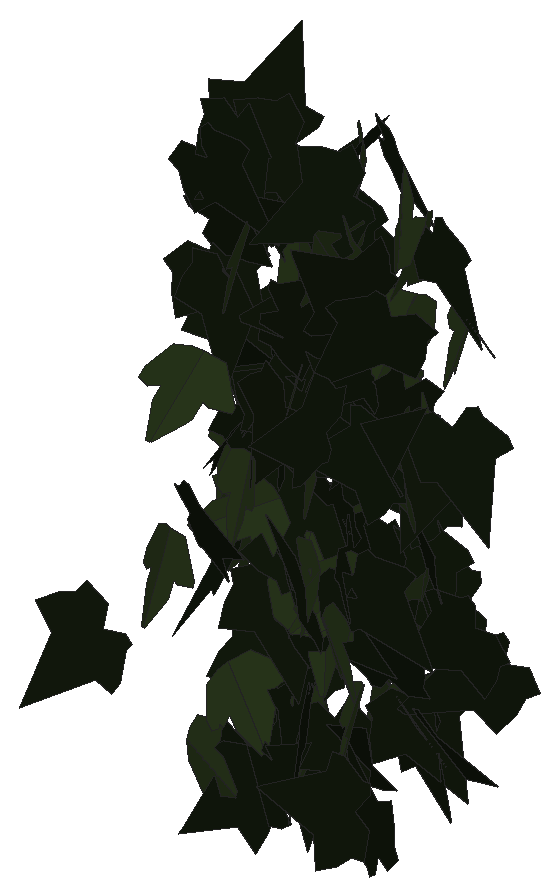
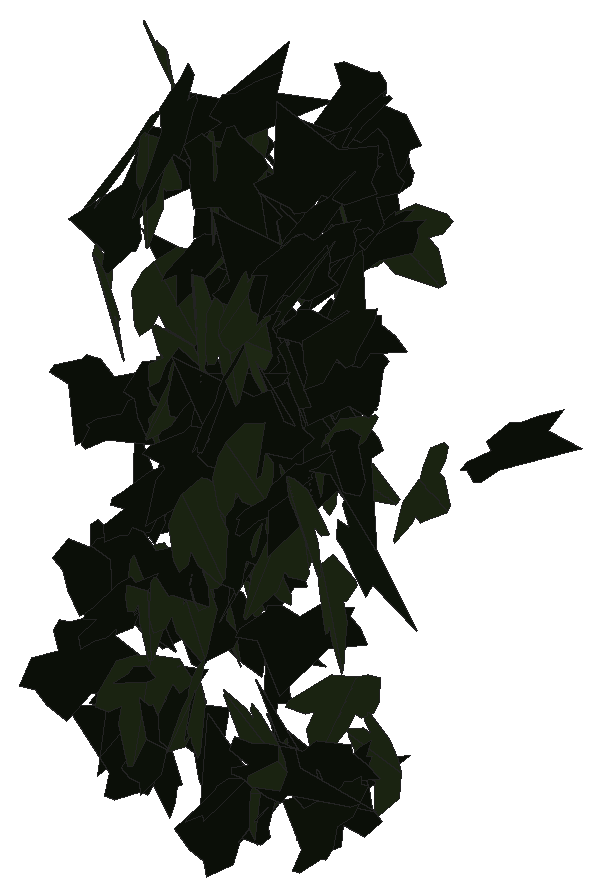
# SketchUp Ruby script. Lengths in inches.
U = 1.inch
M = Sketchup.active_model
def pt(a) = Geom::Point3d.new(a.map { |v| v * U })
def face(e, loops, mat)
  f = e.add_face(loops[0].map { |a| pt(a) })
  loops[1..].each { |l| e.add_face(l.map { |a| pt(a) }).erase! }
  f.material = f.back_material = mat if mat
  f
end
# faces: each face lists its corners as indices into pts; further lists are holes
def faces(e, pts, list, mat = nil) = list.each { |f| face(e, (f[0].is_a?(Array) ? f : [f]).map { |l| l.map { |i| pts[i] } }, mat) }
# xy, xz, yz: faces in a plane at the given z, y or x. An outline is a flat list of corners, or four numbers for a rectangle; further outlines are holes
def ring(l) = l.size == 4 ? [[l[0], l[1]], [l[2], l[1]], [l[2], l[3]], [l[0], l[3]]] : l.each_slice(2).to_a
def flat(e, list, mat, &to3) = list.each { |f| face(e, (f[0].is_a?(Array) ? f : [f]).map { |l| ring(l).map { |u, v| to3.(u, v) } }, mat) }
def xy(e, z, list, mat = nil) = flat(e, list, mat) { |x, y| [x, y, z] }
def xz(e, y, list, mat = nil) = flat(e, list, mat) { |x, z| [x, y, z] }
def yz(e, x, list, mat = nil) = flat(e, list, mat) { |y, z| [x, y, z] }
def lines(e, pts, list) = list.each { |a, b| e.add_line(pt(pts[a]), pt(pts[b])) }
# prism: a flat outline (further loops are holes) pulled along v
def prism(e, loops, v, mat = nil)
  f = face(e, loops, mat); d = Geom::Vector3d.new(v.map { |x| x * U })
  f.pushpull(f.normal.samedirection?(d) ? d.length : -d.length)
end
def box(e, o, s, mat = nil) = prism(e, [[o, [o[0] + s[0], o[1], o[2]], [o[0] + s[0], o[1] + s[1], o[2]], [o[0], o[1] + s[1], o[2]]]], [0, 0, s[2]], mat)
def at(x, y, z, deg = 0) = Geom::Transformation.translation(pt([x, y, z])) * Geom::Transformation.rotation(ORIGIN, Z_AXIS, deg.degrees)
def axes(o, x, y, z) = Geom::Transformation.new([*x, 0, *y, 0, *z, 0, *pt(o).to_a, 1])
def part(name) = M.definitions.add(name)
# library, detail: a bought-in or finely detailed component or shape, given as its bounding box
def library(name, o, s) = part(name).tap { |d| box(d.entities, o, s) }
def detail(e, o, s) = box(e.add_group.entities, o, s)
def put(e, d, t, mat = nil) = e.add_instance(d, t).tap { |i| i.material = mat if mat }
def group(e, t, mat = nil) = e.add_group.tap { |g| g.transformation = t; g.material = mat if mat }.entities
root = M.entities
M.materials.add("efeu1").color = [18, 25, 13]
M.materials.add("efeu2").color = [43, 57, 29]
c1 = part("ivyleaf_10")
p = [[0,0.5,-0.03],[-0.0625,2.02,-0.43],[-0.19,2.01,-0.46],[-0.54,1.05,-0.29],[-0.52,0.625,-0.18],[-0.83,0.76,-0.28],
  [-1.16,0.64,-0.33],[-1.15,0.33,-0.24],[-0.77,-0.39,0.02],[-0.3,-0.51,0.16],[0.04,-0.48,0.23],[-0.02,2.01,-0.4375],
  [-0.06,2.01,-0.43],[0.04,-0.49,0.23],[0.67,-0.49,0.14],[1.38,0.36,-0.2],[1.375,0.51,-0.24],[0.81,0.65,-0.19],
  [0.62,0.59,-0.15],[0.6,1.09,-0.28],[0.5,1.23,-0.31]]
faces(c1.entities,p,[[0,1,2,3,4,5,6,7,8,9,10],[11,12,0,13,14,15,16,17,18,19,20]],"efeu2")
c2 = part("ivyleaf_9")
p = [[1.54,2.16,1.25],[1.36,2.04,1.19],[-0.21,0.99,0.68],[-0.71,1.11,0.82],[-0.85,0.86,0.67],[-0.8,0.17,0.21],
  [-0.9,-0.01,0.1],[-0.67,-0.16,-0.02],[-0.08,-0.08,-0.05],[-0.03,-0.6,-0.4],[0.65,-0.88,-0.66],[0.83,-0.6,-0.49],
  [1.29,-0.42,-0.43],[1.8125,-0.07,-0.26],[1.21,0.44,0.15]]
faces(c2.entities,p,[[0,1,2,3,4,5,6,7,8,9,10,11,12,13,14]],"efeu1")
put(root,c1,axes([32.31,222.57,218.74],[0.42395,-0.25551,-0.07061],[-0.0561,0.04368,-0.49492],[0.25908,0.42756,0.00837]))
put(root,c2,axes([32.14,222.04,220.38],[0.40377,-0.26731,-0.12456],[0.10558,-0.06616,0.48423],[-0.27536,-0.41734,0.00302]))
put(root,c2,axes([32.25,222.2,222.53],[-0.31553,-0.10498,0.37339],[0.37174,0.05553,0.32974],[-0.1107,0.48569,0.043]))
put(root,c2,axes([31.98,222.29,214.44],[0.21673,-0.35207,0.2812],[0.19342,-0.20914,-0.41092],[0.40696,0.28689,0.04554]))
put(root,c2,axes([32.16,222.17,222.4375],[0.07076,-0.49493,-0.00612],[-0.00103,0.00604,-0.49996],[0.49497,0.07077,-0.00016]))
put(root,c1,axes([32.39,221.875,217.21],[0.17943,-0.46368,-0.05301],[-0.01066,0.05271,-0.4971],[0.46658,0.17952,0.00903]))
put(root,c2,axes([32.23,222.39,221.93],[0.08557,-0.40622,-0.27869],[-0.00917,0.2815,-0.41313],[0.49254,0.07582,0.04072]))
put(root,c2,axes([32.81,222.71,215.1],[-0.40746,0.01612,0.28934],[-0.28964,-0.00698,-0.4075],[-0.0091,-0.49969,0.01503]))
put(root,c2,axes([32.39,222.33,215.23],[-0.29931,-0.3482,-0.19791],[0.138,0.14228,-0.45903],[0.37599,-0.32941,0.01094]))
put(root,c2,axes([32.67,221.375,218.97],[-0.19348,0.45479,-0.07573],[0.03096,-0.06913,-0.49423],[-0.46001,-0.19593,-0.00141]))
put(root,c1,axes([32.5,220.06,217.7],[0.00601,0.3694,-0.3369],[-0.01379,-0.33668,-0.3694],[-0.49977,0.01374,0.00614]))
put(root,c1,axes([32.52,221.59,218.74],[0.02832,-0.40737,0.28853],[0.10403,-0.27783,-0.40248],[0.48824,0.08283,0.06902]))
put(root,c2,axes([32.3,222.3,221.5],[0.26872,-0.4191,0.04638],[0.02591,-0.03848,-0.49784],[0.42086,0.26996,0.00104]))
put(root,c2,axes([32.74,221.02,217.41],[-0.38451,0.23721,-0.21419],[0.1678,-0.13536,-0.45113],[-0.27202,-0.41882,0.02448]))
put(root,c2,axes([32.52,221.64,220.46],[-0.28739,-0.3412,-0.2258],[0.14796,0.17059,-0.4461],[0.38146,-0.32323,0.00292]))
put(root,c2,axes([32.41,221.55,222.97],[0.10522,-0.48799,-0.02811],[-0.00403,0.02789,-0.49921],[0.48879,0.10528,0.00194]))
put(root,c2,axes([32.42,221.02,221.34],[0.09643,-0.3928,-0.29395],[0.0414,0.30502,-0.39402],[0.48886,0.05164,0.09135]))
put(root,c2,axes([32.79,222.09,222.54],[-0.27331,-0.26526,0.32394],[-0.19453,-0.2621,-0.37876],[0.37075,-0.33307,0.04007]))
put(root,c2,axes([32.74,218.43,217.34],[-0.25405,-0.35079,0.24981],[-0.12884,-0.21485,-0.43272],[0.41092,-0.28423,0.01878]))
put(root,c2,axes([32.65,221.7,218.95],[0.32197,0.38223,-0.01537],[-0.01291,-0.00921,-0.49975],[-0.38232,0.3222,0.00394]))
put(root,c2,axes([32.62,222.67,218.64],[-0.11973,-0.44473,0.19464],[-0.04975,-0.18817,-0.46056],[0.4829,-0.12966,0.00081]))
put(root,c1,axes([32.36,220.875,214.47],[-0.0658,0.03506,-0.49441],[0.38456,-0.31105,-0.07324],[-0.31271,-0.3899,0.01397]))
put(root,c2,axes([32.63,221.2,219.87],[0.38078,0.30351,0.11352],[0.08986,0.06939,-0.48694],[-0.31134,0.39123,-0.00171]))
put(root,c1,axes([32.7,221.16,215.42],[0.16282,0.44771,0.15182],[0.05846,0.14027,-0.47635],[-0.46912,0.17287,-0.00667]))
put(root,c2,axes([32.68,222.38,221.16],[-0.25046,-0.03882,0.431],[0.42418,0.07655,0.25339],[-0.08566,0.49258,-0.00541]))
put(root,c2,axes([32.49,220.79,222.9],[-0.03863,-0.0412,-0.4968],[0.42177,0.26292,-0.0546],[0.26574,-0.42329,0.01444]))
put(root,c2,axes([32.68,220.99,221.08],[0.02357,-0.49467,0.0689],[0.00007,-0.06897,-0.49522],[0.49944,0.02335,-0.00318]))
put(root,c2,axes([32.46,221.01,221.875],[0.41676,0.08791,-0.26188],[0.21045,0.20601,0.40407],[0.17895,-0.44702,0.13471]))
put(root,c1,axes([32.52,222.78,215.36],[0.13292,-0.09911,-0.47171],[0.39947,-0.25118,0.16533],[-0.26974,-0.42082,0.01241]))
put(root,c1,axes([32.87,222.9375,219.17],[-0.05063,-0.40683,0.28623],[0.09792,-0.29023,-0.39519],[0.4877,0.01604,0.10906]))
put(root,c2,axes([32.87,221.27,214.07],[0.10576,-0.22487,-0.43388],[0.18999,-0.39008,0.24848],[-0.45024,-0.21742,0.00294]))
put(root,c2,axes([32.76,221.72,214.36],[-0.19706,0.29241,0.35449],[0.20982,-0.2859,0.35247],[0.40883,0.28768,-0.01003]))
put(root,c1,axes([32.9,222.95,220.95],[-0.11769,0.21611,0.43525],[0.15057,-0.40958,0.24407],[0.46204,0.18852,0.03133]))
put(root,c2,axes([33.17,221.32,219.67],[-0.31568,0.37174,-0.11028],[0.07145,-0.08401,-0.48769],[-0.38111,-0.32366,-0.00008]))
put(root,c2,axes([32.6875,221.3,213.82],[-0.10946,0.06519,0.4835],[0.39718,-0.27584,0.12711],[0.28331,0.4119,0.00861]))
put(root,c1,axes([32.95,220.97,221.85],[0.26181,-0.40818,0.12186],[0.06481,-0.1032,-0.48492],[0.42102,0.26971,-0.00113]))
put(root,c1,axes([33.28,220.89,218.21],[0.25599,0.03919,-0.42771],[-0.4265,-0.03557,-0.25853],[-0.05069,0.49719,0.01521]))
put(root,c2,axes([33.37,222.06,219.75],[-0.28091,0.07538,-0.40671],[-0.40972,0.01678,0.28609],[0.05678,0.494,0.05234]))
put(root,c2,axes([33.16,221.37,218.43],[0.07392,-0.04564,0.4924],[-0.07408,0.49123,0.05665],[-0.48893,-0.08133,0.06586]))
put(root,c2,axes([32.89,221.78,216.5625],[-0.17419,-0.38433,-0.26823],[0.11242,0.24355,-0.42196],[0.45499,-0.20731,0.00156]))
put(root,c1,axes([33.04,221.94,217.66],[-0.02961,-0.35779,-0.34801],[0.06373,0.34305,-0.35812],[0.49504,-0.06557,0.02528]))
put(root,c1,axes([33.17,219.71,220.58],[0.32097,0.28919,-0.25169],[-0.18565,-0.16996,-0.43203],[-0.33543,0.37079,-0.00173]))
put(root,c2,axes([32.82,222.56,219.15],[-0.10704,-0.01487,0.48818],[0.48028,-0.09402,0.10244],[0.08875,0.49086,0.03441]))
put(root,c1,axes([33.01,222.33,214.49],[-0.00134,-0.22121,0.4484],[0.26873,-0.37845,-0.1859],[0.42164,0.2405,0.11991]))
put(root,c1,axes([33.24,222.66,220.74],[0.02883,-0.49844,-0.02702],[0.00013,0.02708,-0.49927],[0.49917,0.02878,0.00169]))
put(root,c2,axes([32.96,221.12,219.38],[0.04144,0.01784,-0.49796],[0.19221,0.46043,0.03249],[0.45971,-0.19412,0.03131]))
put(root,c1,axes([33.06,222.41,220.36],[0.17276,-0.21031,0.41943],[0.27027,-0.32076,-0.27216],[0.38355,0.32075,0.00285]))
put(root,c2,axes([33.05,222.09,214.25],[0.07021,-0.47379,0.1435],[0.01954,-0.14217,-0.47896],[0.49466,0.07287,-0.00144]))
put(root,c2,axes([33.125,222.98,219.84],[0.14798,-0.14163,-0.45612],[0.34089,-0.30312,0.20472],[-0.3345,-0.37157,0.00685]))
put(root,c2,axes([33.56,222.35,222.61],[-0.21193,0.42636,-0.15265],[0.04814,-0.14637,-0.47567],[-0.4503,-0.21632,0.02099]))
put(root,c1,axes([33.15,221.76,221.23],[0.31977,-0.13647,0.35933],[0.33699,-0.12529,-0.34747],[0.18489,0.46441,0.01185]))
put(root,c2,axes([33.4375,221.26,219.4],[-0.3062,-0.19412,0.34433],[0.31058,0.15127,0.36147],[-0.24451,0.43524,0.02794]))
put(root,c2,axes([33.78,222.56,219.21],[0.04114,-0.00309,0.4983],[-0.47583,0.14823,0.0402],[-0.14797,-0.47751,0.00926]))
put(root,c2,axes([33.1875,222.39,217.54],[0.0497,-0.17552,0.46553],[0.18697,-0.42697,-0.18094],[0.46106,0.19207,0.0232]))
put(root,c2,axes([33.2,222.5,214],[0.48721,-0.04367,-0.10352],[0.10669,0.0354,0.4872],[-0.03522,-0.49683,0.04381]))
put(root,c2,axes([33.33,222.3,214.55],[0.07332,-0.47465,-0.13904],[-0.00083,0.14044,-0.47987],[0.49459,0.0706,0.01981]))
put(root,c1,axes([33.59,221.29,220.23],[0.28433,-0.40044,-0.09383],[-0.04158,0.0855,-0.49088],[0.40918,0.28695,0.01532]))
put(root,c2,axes([33.83,221.67,217.66],[0.06786,-0.08371,0.48825],[-0.29047,0.39247,0.10766],[-0.40127,-0.29826,0.00463]))
put(root,c1,axes([33.7,222.33,222.5],[0.17303,-0.29338,-0.36604],[-0.13695,0.34156,-0.3385],[0.44867,0.2174,0.03784]))
put(root,c2,axes([33.46,221.46,217.53],[0.28464,-0.29456,-0.28674],[-0.18888,0.21605,-0.40945],[0.36511,0.34141,0.01172]))
put(root,c2,axes([33.82,221.25,217.57],[-0.37351,-0.32309,0.07815],[0.0608,0.04916,0.49385],[-0.3268,0.37842,0.00256]))
put(root,c1,axes([33.69,222.71,218.0625],[-0.00727,-0.46456,0.18474],[0.02734,-0.18486,-0.46377],[0.4992,0.00336,0.02809]))
put(root,c2,axes([33.9,222.48,218.6875],[-0.08354,-0.059,0.48943],[-0.40051,-0.2813,-0.10227],[0.28742,-0.40913,-0.00027]))
put(root,c2,axes([33.57,222.54,218.91],[-0.02965,-0.31912,-0.38377],[0.10077,0.37271,-0.31771],[0.48884,-0.09619,0.04221]))
put(root,c1,axes([33.92,222.35,220.7],[0.16493,-0.37373,-0.28832],[-0.11145,0.26594,-0.40848],[0.45867,0.19901,0.00442]))
put(root,c2,axes([34.23,221.16,221.14],[-0.09751,-0.09507,-0.4811],[-0.3884,-0.2845,0.13494],[-0.2994,0.40003,-0.01837]))
put(root,c2,axes([33.6,222.01,221.98],[-0.16548,-0.17035,-0.44],[0.39379,0.20697,-0.22823],[0.25989,-0.42207,0.06566]))
put(root,c1,axes([33.8,221.05,216.83],[0.49694,0.05359,-0.01355],[0.0134,0.00209,0.49982],[0.05363,-0.49712,0.00064]))
put(root,c2,axes([33.74,220.77,219.76],[-0.02738,-0.3822,0.32121],[-0.02304,-0.32038,-0.38318],[0.49872,-0.03579,-0.00006]))
put(root,c1,axes([33.97,222.28,215.42],[0.03969,-0.09222,-0.48982],[-0.0581,0.48716,-0.09643],[0.49502,0.06457,0.02795]))
put(root,c2,axes([33.75,222.25,221.42],[0.10763,-0.45316,-0.18182],[-0.04151,0.17702,-0.46577],[0.48651,0.11535,0.00048]))
put(root,c2,axes([34.11,221.58,222.51],[-0.24259,-0.25155,0.3576],[-0.24036,-0.26488,-0.34938],[0.36521,-0.34142,0.00759]))
put(root,c2,axes([33.83,221.12,215.49],[-0.16354,0.09011,-0.46383],[0.42072,-0.19564,-0.18634],[-0.21507,-0.45123,-0.01183]))
put(root,c1,axes([34.26,221.44,221.93],[-0.35349,0.06178,0.34817],[-0.34555,0.04417,-0.35867],[-0.07507,-0.4942,0.01147]))
put(root,c1,axes([34.15,220.78,217.57],[0.24726,-0.29081,-0.32294],[-0.20999,0.24535,-0.38172],[0.38048,0.3244,-0.00081]))
put(root,c2,axes([34.09,220.91,217.01],[0.13871,-0.42886,0.21642],[-0.02741,0.21783,0.44922],[-0.47959,-0.13649,0.03693]))
put(root,c2,axes([33.59,220.9375,220.98],[0.19162,-0.01967,-0.46141],[0.39057,0.27347,0.15055],[0.24644,-0.41812,0.12017]))
put(root,c1,axes([33.94,219.72,219.41],[0.41322,-0.26508,0.09477],[0.08082,-0.04953,-0.49093],[0.26966,0.42104,0.00192]))
put(root,c1,axes([34.17,222.3,219.48],[0.03638,-0.14598,-0.47683],[-0.01439,0.47759,-0.14731],[0.49847,0.02444,0.03055]))
put(root,c1,axes([33.96,221.26,216.78],[0.46324,-0.09978,0.15954],[0.15524,-0.03694,-0.47385],[0.10634,0.48855,-0.00324]))
put(root,c1,axes([34.08,221.38,221.65],[-0.08067,-0.37345,-0.32253],[-0.0126,-0.32515,0.37963],[-0.49329,0.06938,0.04305]))
put(root,c1,axes([33.83,222.52,219.72],[0.28334,0.0399,0.41003],[0.39739,0.10472,-0.2848],[-0.10861,0.48728,0.02763]))
put(root,c2,axes([33.83,221.125,216.93],[0.0591,-0.02817,-0.4957],[0.40425,0.29255,0.03157],[0.28825,-0.4045,0.05735]))
put(root,c2,axes([34.26,221.41,217.72],[0.20083,-0.1407,-0.43574],[-0.34872,0.26137,-0.24512],[0.29676,0.40235,0.00685]))
put(root,c1,axes([34.3,222.18,216.76],[-0.11806,-0.47316,0.11038],[-0.0201,-0.10874,-0.48762],[0.48545,-0.11957,0.00666]))
put(root,c2,axes([34.39,222.99,218.02],[-0.01171,-0.37473,-0.33082],[-0.00935,-0.33069,0.37491],[-0.49978,0.01497,0.00074]))
put(root,c1,axes([34.42,221.37,217.33],[0.23199,0.1961,-0.39715],[-0.29803,-0.26254,-0.30372],[-0.32765,0.37765,-0.00493]))
put(root,c2,axes([34.1,221.71,220.25],[-0.04526,-0.30569,0.39307],[0.0491,-0.39551,-0.30193],[0.49552,0.01127,0.06582]))
put(root,c2,axes([34.2,222.23,222.97],[0.39088,-0.15568,-0.27014],[-0.24935,0.10397,-0.42073],[0.18717,0.46363,0.00364]))
put(root,c1,axes([34.1,222.06,216.86],[-0.05364,0.04323,0.49523],[0.30389,-0.39135,0.06708],[0.39341,0.30819,0.01571]))
put(root,c2,axes([34.41,222.25,219.57],[-0.04171,0.14428,-0.47691],[0.13304,-0.45798,-0.15019],[-0.48017,-0.13943,-0.00018]))
put(root,c1,axes([34.4,222.35,220.68],[-0.17357,-0.40716,0.23258],[0.01817,-0.25365,-0.4305],[0.46856,-0.14099,0.10285]))
put(root,c2,axes([34.35,222.32,217.07],[-0.14554,-0.20553,0.43194],[-0.04227,-0.4442,-0.2256],[0.47648,-0.10219,0.11192]))
put(root,c2,axes([34.5,221.85,215.84],[0.34238,-0.16847,0.32311],[-0.28135,0.15953,0.38131],[-0.23157,-0.44291,0.01445]))
put(root,c2,axes([34.12,222.67,214.9],[0.38713,-0.11578,-0.29449],[0.28137,-0.08694,0.40407],[-0.14477,-0.47858,-0.00216]))
put(root,c1,axes([34.34,220.8,219.59],[0.1682,-0.37429,0.28569],[0.17293,-0.23306,-0.40716],[0.43795,0.23578,0.05105]))
put(root,c1,axes([34.375,222.17,218.5625],[0.16129,-0.45177,-0.14102],[0.04778,-0.13268,0.4797],[-0.47085,-0.16821,0.00037]))
put(root,c1,axes([34.57,222.41,216.89],[0.02054,-0.48637,-0.11413],[-0.00976,0.11382,-0.48678],[0.49948,0.02222,-0.00482]))
put(root,c2,axes([34.34,222.58,217.26],[-0.19721,-0.246,-0.38806],[0.26026,0.28821,-0.31496],[0.37865,-0.32622,0.01437]))
put(root,c2,axes([34.27,222.625,214.86],[-0.08518,-0.04186,-0.49091],[0.48583,0.07574,-0.09076],[0.08196,-0.49246,0.02777]))
put(root,c1,axes([34.63,222.36,215.44],[-0.32174,-0.37256,-0.08767],[0.05604,0.06744,-0.49225],[0.37861,-0.32658,-0.00164]))
put(root,c2,axes([34.79,222.98,216.46],[0.01335,-0.4207,-0.26987],[0.00931,-0.26971,0.42091],[-0.49973,-0.01627,0.00063]))
put(root,c2,axes([34.79,220.87,221.57],[0.11067,0.10687,0.47574],[-0.37505,-0.29309,0.15309],[0.31159,-0.39074,0.01529]))
put(root,c2,axes([34.92,221.11,213.86],[0.10325,-0.08462,0.48185],[-0.2244,0.42941,0.12349],[-0.43473,-0.24175,0.05069]))
put(root,c1,axes([34.66,221,215.86],[0.30377,-0.36777,0.14991],[0.09643,-0.11478,-0.477],[0.38526,0.3187,0.00119]))
put(root,c2,axes([34.62,222.24,215.33],[-0.01406,-0.34104,-0.36537],[0.01025,0.36524,-0.34131],[0.4997,-0.01709,-0.00328]))
put(root,c1,axes([34.89,221.96,221.93],[0.06806,-0.41447,-0.27127],[-0.0637,0.26422,-0.41968],[0.49123,0.09169,-0.01683]))
put(root,c2,axes([34.82,222.54,218.875],[-0.21094,-0.44896,0.06278],[-0.01686,-0.06143,-0.49593],[0.45301,-0.21134,0.01077]))
put(root,c2,axes([34.61,222.39,217.39],[-0.01201,-0.07695,0.4939],[0.16346,-0.46748,-0.06886],[0.47237,0.15981,0.03639]))
put(root,c2,axes([34.47,222.55,214.59],[0.22366,-0.19528,0.4023],[0.32977,-0.23178,-0.29585],[0.30204,0.39767,0.02511]))
put(root,c2,axes([34.61,221.11,217.53],[-0.08476,-0.12739,-0.47601],[0.28675,0.38005,-0.15277],[0.40074,-0.29889,0.00863]))
put(root,c2,axes([35.34,220.09,215],[-0.21543,-0.11127,-0.43728],[-0.39281,-0.19218,0.24242],[-0.22202,0.44798,-0.00461]))
put(root,c1,axes([34.98,221.53,218.58],[-0.44273,0.20194,0.11496],[0.10365,-0.04978,0.4866],[0.20797,0.45469,0.00222]))
put(root,c2,axes([34.6,217.9375,219.8125],[0.30761,-0.05421,-0.39044],[0.39394,0.02487,0.30691],[-0.01385,-0.49643,0.05801]))
put(root,c1,axes([35.07,222.61,220.63],[0.3208,-0.37732,-0.06869],[-0.04371,0.053,-0.49526],[0.38103,0.32376,0.00102]))
put(root,c1,axes([34.8125,220.4,217.1875],[-0.17128,0.18285,-0.4327],[0.28486,-0.32579,-0.25043],[-0.37352,-0.3323,0.00743]))
put(root,c2,axes([34.79,220.64,219.3],[-0.1401,0.04158,0.47817],[0.46816,-0.098,0.14569],[0.10584,0.48854,-0.01148]))
put(root,c2,axes([34.77,222.39,221.375],[0.31985,-0.31081,0.22604],[0.15915,-0.16057,-0.44597],[0.34981,0.35723,-0.00378]))
put(root,c2,axes([35.33,220.82,221.55],[0.05469,0.1434,-0.47586],[-0.15969,-0.44828,-0.15344],[-0.47065,0.16876,-0.00324]))
put(root,c2,axes([35.36,222.96,215.78],[-0.06446,-0.04211,-0.49404],[-0.09373,-0.48818,0.05384],[-0.48689,0.09956,0.05504]))
put(root,c2,axes([35.2,220.87,219.55],[0.10705,-0.40414,-0.27424],[0.07394,-0.2641,0.41807],[-0.48278,-0.13007,0.00322]))
put(root,c2,axes([35.55,219.27,220.73],[-0.37515,0.26869,0.19253],[-0.15449,0.11495,-0.46143],[-0.29223,-0.4057,-0.00323]))
put(root,c1,axes([35.32,221.125,222.4],[0.34916,-0.18984,0.30339],[-0.2504,0.17325,0.39659],[-0.2557,-0.42889,0.02591]))
put(root,c2,axes([35.54,222.2,216.69],[0.05086,0.04784,-0.4951],[-0.40404,-0.2863,-0.06917],[-0.29012,0.40711,0.00954]))
put(root,c2,axes([35.04,222.1,222.02],[0.27918,-0.41147,-0.05247],[-0.03112,0.0423,-0.49723],[0.41363,0.2809,-0.00199]))
put(root,c2,axes([35.08,222.42,219.1875],[-0.19035,-0.27495,-0.37171],[0.26768,0.26222,-0.33104],[0.37698,-0.32502,0.04737]))
